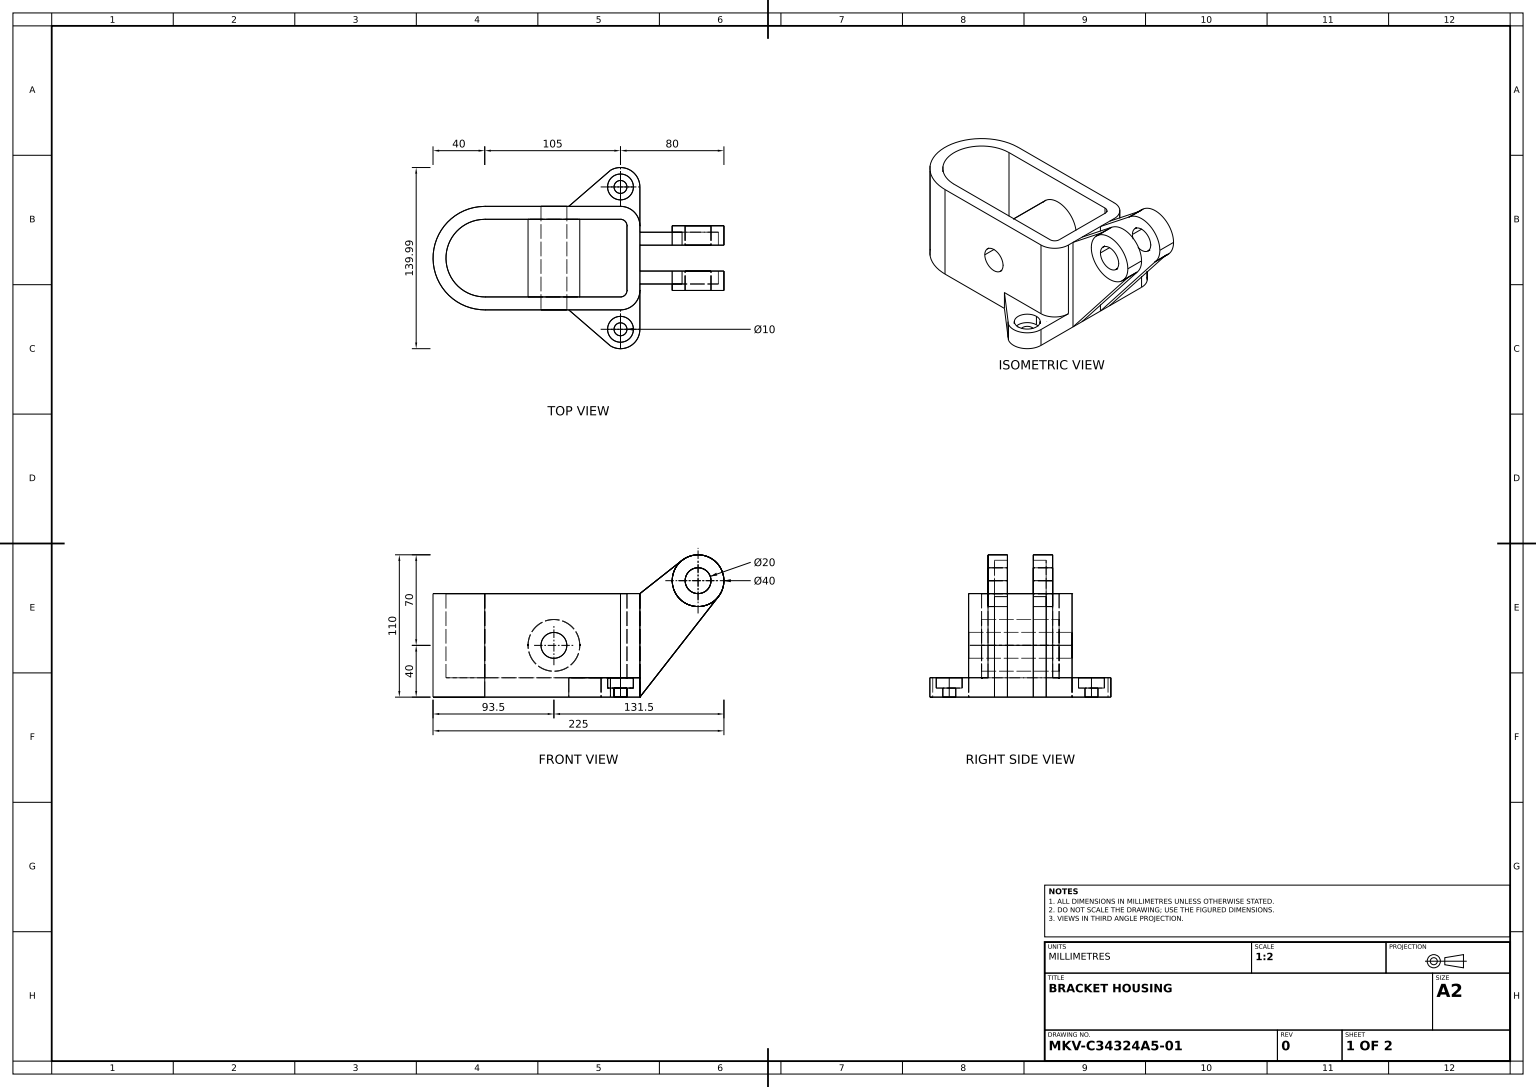
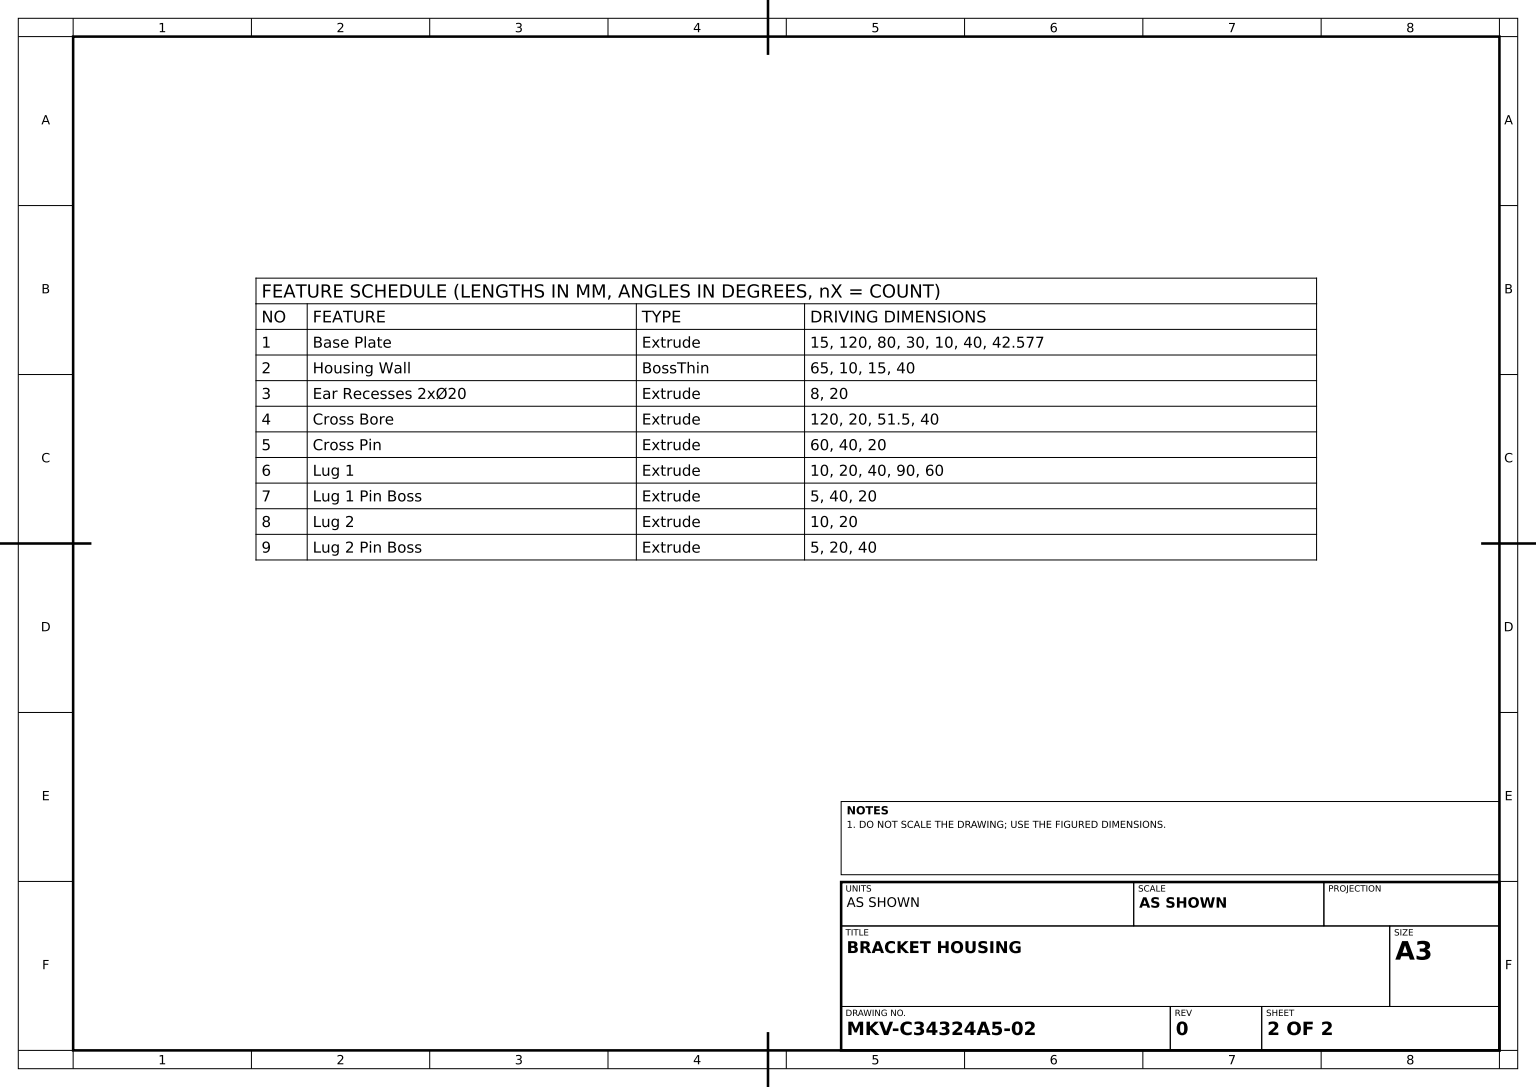
solid
v1 (85,90,20)
v2 (120.753851,77.67863,20)
e1 v1 v2 CIRCLE(AX(P(105,90,20),D(0,0,1),D(1,0,0)),20)
v3 (120.753851,77.67863,10)
e2 v2 v3 LINE
v4 (125,90,10)
e3 v3 v4 CIRCLE(AX(P(105,90,10),D(0,0,1),D(1,0,0)),20)
v5 (125,90,25)
e4 v5 v4 LINE
v6 (85,90,25)
e5 v6 v5 CIRCLE(AX(P(105,90,25),D(0,0,1),D(1,0,0)),20)
e6 v6 v1 LINE
face CYL(AX(P(105,90,20),D(0,0,-1),D(-1,0,0)),20) [e1 e2 e3 -e4 -e5 e6]
v7 (45,15,30)
v8 (50,15,25)
e7 v7 v8 CIRCLE(AX(P(45,15,25),D(0,1,0),D(1,0,0)),5)
v9 (45,80,30)
e8 v9 v7 LINE
v10 (50,80,25)
e9 v9 v10 CIRCLE(AX(P(45,80,25),D(0,1,0),D(1,0,0)),5)
e10 v10 v8 LINE
face CYL(AX(P(45,80,25),D(0,-1,0),D(0,0,-1)),5) rev [-e7 -e8 e9 e10]
v11 (5,15,40)
v12 (5,0,40)
e11 v11 v12 LINE
v13 (37.224741,0,67.827523)
e12 v12 v13 LINE
v14 (37.224741,15,67.827523)
e13 v14 v13 LINE
e14 v11 v14 LINE
face PLANE(AX(P(-17.650842,15,20.439972),D(0.653580385,0,-0.756857107),D(-0.756857107,0,-0.653580385))) rev [e11 e12 -e13 -e14]
v15 (45,0,-50)
v16 (45,0,-60)
e15 v15 v16 CIRCLE(AX(P(45,0,-55),D(0,1,0),D(0,0,1)),5)
e16 v16 v15 CIRCLE(AX(P(45,0,-55),D(0,1,0),D(0,0,1)),5)
v17 (45,0,60)
v18 (45,0,50)
e17 v17 v18 CIRCLE(AX(P(45,0,55),D(0,1,0),D(0,0,1)),5)
e18 v18 v17 CIRCLE(AX(P(45,0,55),D(0,1,0),D(0,0,1)),5)
v19 (-60,0,-40)
v20 (5,0,-40)
e19 v19 v20 LINE
v21 (37.224741,0,-67.827523)
e20 v20 v21 LINE
v22 (45,0,-70)
e21 v22 v21 CIRCLE(AX(P(45,0,-55),D(0,1,0),D(0,0,1)),15)
v23 (60,0,-55)
e22 v23 v22 CIRCLE(AX(P(45,0,-55),D(0,1,0),D(0,0,1)),15)
v24 (60,0,-20)
e23 v24 v23 LINE
v25 (60,0,-10)
e24 v24 v25 LINE
v26 (60,0,10)
e25 v26 v25 LINE
v27 (60,0,20)
e26 v27 v26 LINE
v28 (60,0,55)
e27 v28 v27 LINE
e28 v13 v28 CIRCLE(AX(P(45,0,55),D(0,1,0),D(0,0,1)),15)
v29 (-60,0,40)
e29 v29 v12 LINE
e30 v19 v29 CIRCLE(AX(P(-60,0,0),D(0,1,0),D(0,0,1)),40)
face PLANE(AX(P(0,0,0),D(0,1,0),D(0,0,1))) rev [e15 e16] [e17 e18] [e19 e20 -e21 -e22 -e23 e24 -e25 -e26 -e27 -e28 -e12 -e29 -e30]
v30 (45,7,-45)
v31 (45,15,-45)
e31 v30 v31 LINE
v32 (45,15,-65)
e32 v31 v32 CIRCLE(AX(P(45,15,-55),D(0,1,0),D(0,0,1)),10)
v33 (45,7,-65)
e33 v33 v32 LINE
e34 v30 v33 CIRCLE(AX(P(45,7,-55),D(0,1,0),D(0,0,1)),10)
face CYL(AX(P(45,7,-55),D(0,1,0),D(0,0,1)),10) rev [e31 e32 -e33 -e34]
v34 (95,90,-25)
v35 (115,90,-25)
e35 v34 v35 CIRCLE(AX(P(105,90,-25),D(0,0,-1),D(-1,0,0)),10)
v36 (115,90,-10)
e36 v35 v36 LINE
v37 (95,90,-10)
e37 v36 v37 CIRCLE(AX(P(105,90,-10),D(0,0,1),D(1,0,0)),10)
e38 v34 v37 LINE
face CYL(AX(P(105,90,-20),D(0,0,1),D(1,0,0)),10) rev [e35 e36 e37 -e38]
v38 (3.5,40,40)
v39 (-16.5,40,40)
e39 v38 v39 CIRCLE(AX(P(-6.5,40,40),D(0,0,1),D(1,0,0)),10)
e40 v39 v38 CIRCLE(AX(P(-6.5,40,40),D(0,0,1),D(1,0,0)),10)
v40 (45,15,40)
e41 v11 v40 LINE
v41 (45,80,40)
e42 v41 v40 LINE
v42 (-60,80,40)
e43 v42 v41 LINE
e44 v42 v29 LINE
face PLANE(AX(P(0,15,40),D(0,0,-1),D(-1,0,0))) rev [-e39 -e40] [e29 -e11 e41 -e42 -e43 e44]
v43 (3.5,40,-40)
v44 (-16.5,40,-40)
e45 v43 v44 CIRCLE(AX(P(-6.5,40,-40),D(0,0,-1),D(-1,0,0)),10)
e46 v44 v43 CIRCLE(AX(P(-6.5,40,-40),D(0,0,-1),D(-1,0,0)),10)
v45 (-60,80,-40)
e47 v45 v19 LINE
v46 (45,80,-40)
e48 v46 v45 LINE
v47 (45,15,-40)
e49 v46 v47 LINE
v48 (5,15,-40)
e50 v47 v48 LINE
e51 v48 v20 LINE
face PLANE(AX(P(0,15,-40),D(0,0,-1),D(-1,0,0))) [-e45 -e46] [-e19 -e47 -e48 e49 e50 e51]
v49 (120.753851,77.67863,-10)
v50 (125,90,-10)
e52 v49 v50 CIRCLE(AX(P(105,90,-10),D(0,0,1),D(1,0,0)),20)
v51 (120.753851,77.67863,-20)
e53 v51 v49 LINE
v52 (85,90,-20)
e54 v51 v52 CIRCLE(AX(P(105,90,-20),D(0,0,-1),D(1,0,0)),20)
v53 (85,90,-25)
e55 v53 v52 LINE
v54 (125,90,-25)
e56 v54 v53 CIRCLE(AX(P(105,90,-25),D(0,0,-1),D(-1,0,0)),20)
e57 v54 v50 LINE
face CYL(AX(P(105,90,-20),D(0,0,1),D(1,0,0)),20) [-e52 -e53 e54 -e55 -e56 e57]
v55 (13.5,40,30)
v56 (-26.5,40,30)
e58 v55 v56 CIRCLE(AX(P(-6.5,40,30),D(0,0,1),D(1,0,0)),20)
v57 (13.5,40,-30)
e59 v55 v57 LINE
v58 (-26.5,40,-30)
e60 v57 v58 CIRCLE(AX(P(-6.5,40,-30),D(0,0,1),D(1,0,0)),20)
e61 v56 v58 LINE
face CYL(AX(P(-6.5,40,30),D(0,0,-1),D(-1,0,0)),20) [-e58 e59 e60 -e61]
v59 (45,7,45)
v60 (45,15,45)
e62 v59 v60 LINE
v61 (45,15,65)
e63 v60 v61 CIRCLE(AX(P(45,15,55),D(0,1,0),D(0,0,1)),10)
v62 (45,7,65)
e64 v62 v61 LINE
e65 v59 v62 CIRCLE(AX(P(45,7,55),D(0,1,0),D(0,0,1)),10)
face CYL(AX(P(45,7,55),D(0,1,0),D(0,0,1)),10) rev [e62 e63 -e64 -e65]
v63 (-60,80,-30)
v64 (-60,80,30)
e66 v63 v64 CIRCLE(AX(P(-60,80,0),D(0,1,0),D(1,0,0)),30)
v65 (-60,15,30)
e67 v64 v65 LINE
v66 (-60,15,-30)
e68 v66 v65 CIRCLE(AX(P(-60,15,0),D(0,1,0),D(1,0,0)),30)
e69 v63 v66 LINE
face CYL(AX(P(-60,80,0),D(0,-1,0),D(0,0,-1)),30) rev [e66 e67 -e68 -e69]
v67 (60,80,-10)
e70 v67 v25 LINE
v68 (60,80,10)
e71 v68 v67 LINE
e72 v68 v26 LINE
face PLANE(AX(P(60,15,0),D(-1,0,0),D(0,0,1))) rev [-e70 -e71 e72 e25]
v69 (60,15,-55)
e73 v69 v23 LINE
v70 (60,15,-25)
e74 v70 v69 LINE
v71 (60,80,-25)
e75 v71 v70 LINE
v72 (60,80,-20)
e76 v72 v71 LINE
e77 v72 v24 LINE
face PLANE(AX(P(60,15,0),D(-1,0,0),D(0,0,1))) rev [-e73 -e74 -e75 -e76 e77 e23]
e78 v65 v7 LINE
v73 (50,15,-25)
e79 v8 v73 LINE
v74 (45,15,-30)
e80 v73 v74 CIRCLE(AX(P(45,15,-25),D(0,1,0),D(1,0,0)),5)
e81 v74 v66 LINE
face PLANE(AX(P(0,15,0),D(0,1,0),D(0,0,1))) [e68 e78 e7 e79 e80 e81]
e82 v70 v47 CIRCLE(AX(P(45,15,-25),D(0,1,0),D(0,0,-1)),15)
v75 (45,15,-70)
e83 v69 v75 CIRCLE(AX(P(45,15,-55),D(0,1,0),D(0,0,1)),15)
v76 (37.224741,15,-67.827523)
e84 v75 v76 CIRCLE(AX(P(45,15,-55),D(0,1,0),D(0,0,1)),15)
e85 v48 v76 LINE
e86 v32 v31 CIRCLE(AX(P(45,15,-55),D(0,1,0),D(0,0,1)),10)
face PLANE(AX(P(0,15,0),D(0,1,0),D(0,0,1))) [-e50 -e82 e74 e83 e84 -e85] [-e86 -e32]
v77 (95,90,10)
v78 (115,90,10)
e87 v77 v78 CIRCLE(AX(P(105,90,10),D(0,0,1),D(1,0,0)),10)
v79 (95,90,25)
e88 v79 v77 LINE
v80 (115,90,25)
e89 v79 v80 CIRCLE(AX(P(105,90,25),D(0,0,1),D(1,0,0)),10)
e90 v80 v78 LINE
face CYL(AX(P(105,90,20),D(0,0,-1),D(-1,0,0)),10) rev [-e87 -e88 e89 e90]
e91 v61 v60 CIRCLE(AX(P(45,15,55),D(0,1,0),D(0,0,1)),10)
e92 v62 v59 CIRCLE(AX(P(45,7,55),D(0,1,0),D(0,0,1)),10)
face CYL(AX(P(45,7,55),D(0,1,0),D(0,0,1)),10) rev [e91 -e62 -e92 e64]
v81 (50,80,-25)
e93 v10 v81 LINE
e94 v81 v73 LINE
face PLANE(AX(P(50,80,25),D(-1,0,0),D(0,0,1))) [-e79 -e10 e93 e94]
e95 v71 v46 CIRCLE(AX(P(45,80,-25),D(0,1,0),D(0,0,-1)),15)
e96 v45 v42 CIRCLE(AX(P(-60,80,0),D(0,1,0),D(0,0,1)),40)
v82 (60,80,25)
e97 v41 v82 CIRCLE(AX(P(45,80,25),D(0,1,0),D(0,0,1)),15)
v83 (60,80,20)
e98 v82 v83 LINE
e99 v83 v68 LINE
e100 v72 v67 LINE
v84 (45,80,-30)
e101 v84 v63 LINE
e102 v81 v84 CIRCLE(AX(P(45,80,-25),D(0,1,0),D(1,0,0)),5)
e103 v64 v9 LINE
face PLANE(AX(P(-60,80,0),D(0,1,0),D(0,0,1))) [e76 e95 e48 e96 e43 e97 e98 e99 e71 -e100] [-e66 -e101 -e102 -e93 -e9 -e103]
e104 v26 v3 LINE
v85 (92.620412,105.708145,10)
e105 v68 v85 LINE
e106 v4 v85 CIRCLE(AX(P(105,90,10),D(0,0,1),D(1,0,0)),20)
e107 v78 v77 CIRCLE(AX(P(105,90,10),D(0,0,1),D(1,0,0)),10)
face PLANE(AX(P(0,0,10),D(0,0,1),D(1,0,0))) rev [-e3 -e104 -e72 e105 -e106] [e87 e107]
v86 (45,7,-50)
v87 (45,7,-60)
e108 v86 v87 CIRCLE(AX(P(45,7,-55),D(0,1,0),D(0,0,1)),5)
e109 v87 v16 LINE
e110 v86 v15 LINE
face CYL(AX(P(45,15,-55),D(0,-1,0),D(0,0,-1)),5) rev [e108 e109 -e15 -e110]
v88 (60,15,55)
v89 (60,15,25)
e111 v88 v89 LINE
e112 v40 v89 CIRCLE(AX(P(45,15,25),D(0,1,0),D(0,0,1)),15)
e113 v14 v88 CIRCLE(AX(P(45,15,55),D(0,1,0),D(0,0,1)),15)
face PLANE(AX(P(0,15,0),D(0,1,0),D(0,0,1))) [e111 -e112 -e41 e14 e113] [-e91 -e63]
e114 v87 v86 CIRCLE(AX(P(45,7,-55),D(0,1,0),D(0,0,1)),5)
e115 v33 v30 CIRCLE(AX(P(45,7,-55),D(0,1,0),D(0,0,1)),10)
face PLANE(AX(P(45,7,-55),D(0,1,0),D(0,0,1))) [-e114 -e108] [e34 e115]
face CYL(AX(P(45,80,-25),D(0,-1,0),D(0,0,-1)),15) [-e49 -e95 e75 e82]
e116 v82 v89 LINE
face CYL(AX(P(45,80,25),D(0,-1,0),D(0,0,-1)),15) [-e116 -e97 e42 e112]
e117 v43 v38 LINE
e118 v44 v39 LINE
face CYL(AX(P(-6.5,40,-80),D(0,0,1),D(1,0,0)),10) rev [-e117 e45 e118 e40]
e119 v58 v57 CIRCLE(AX(P(-6.5,40,-30),D(0,0,1),D(1,0,0)),20)
e120 v84 v74 LINE
face PLANE(AX(P(-60,80,-30),D(0,0,1),D(1,0,0))) [-e60 -e119] [e69 -e81 -e120 e101]
e121 v88 v28 LINE
face CYL(AX(P(45,15,55),D(0,-1,0),D(0,0,-1)),15) [e28 -e121 -e113 e13]
face CYL(AX(P(-60,15,0),D(0,-1,0),D(0,0,-1)),40) [e47 e30 -e44 -e96]
v90 (92.620412,105.708145,20)
e122 v83 v90 LINE
e123 v83 v27 LINE
e124 v27 v2 LINE
e125 v90 v1 CIRCLE(AX(P(105,90,20),D(0,0,1),D(1,0,0)),20)
face PLANE(AX(P(0,0,20),D(0,0,1),D(1,0,0))) [-e122 e123 e124 -e1 -e125]
e126 v35 v34 CIRCLE(AX(P(105,90,-25),D(0,0,-1),D(-1,0,0)),10)
e127 v37 v36 CIRCLE(AX(P(105,90,-10),D(0,0,1),D(1,0,0)),10)
face CYL(AX(P(105,90,-20),D(0,0,1),D(1,0,0)),10) rev [-e36 e126 e38 e127]
v91 (45,7,60)
e128 v91 v17 LINE
v92 (45,7,50)
e129 v92 v18 LINE
e130 v92 v91 CIRCLE(AX(P(45,7,55),D(0,1,0),D(0,0,1)),5)
face CYL(AX(P(45,15,55),D(0,-1,0),D(0,0,-1)),5) rev [e128 -e18 -e129 e130]
e131 v91 v92 CIRCLE(AX(P(45,7,55),D(0,1,0),D(0,0,1)),5)
face PLANE(AX(P(45,7,55),D(0,1,0),D(0,0,1))) [e92 e65] [-e130 -e131]
e132 v25 v49 LINE
e133 v24 v51 LINE
face PLANE(AX(P(37.227576,-29.116355,-20),D(0.787692574,-0.616068509,0),D(0.616068509,0.787692574,0))) [e53 -e132 -e24 e133]
e134 v56 v55 CIRCLE(AX(P(-6.5,40,30),D(0,0,1),D(1,0,0)),20)
face PLANE(AX(P(-60,80,30),D(0,0,-1),D(-1,0,0))) [-e78 -e67 e103 e8] [e134 e58]
v93 (92.620412,105.708145,-20)
e135 v93 v72 LINE
e136 v52 v93 CIRCLE(AX(P(105,90,-20),D(0,0,-1),D(1,0,0)),20)
face PLANE(AX(P(0,0,-20),D(0,0,1),D(1,0,0))) rev [-e133 -e77 -e135 -e136 -e54]
face CYL(AX(P(45,15,-55),D(0,-1,0),D(0,0,-1)),5) rev [-e109 e114 e110 -e16]
e137 v5 v6 CIRCLE(AX(P(105,90,25),D(0,0,1),D(1,0,0)),20)
e138 v80 v79 CIRCLE(AX(P(105,90,25),D(0,0,1),D(1,0,0)),10)
face PLANE(AX(P(105,90,25),D(0,0,1),D(1,0,0))) [e137 e5] [-e89 -e138]
face CYL(AX(P(45,80,-25),D(0,-1,0),D(0,0,-1)),5) rev [e120 -e80 -e94 e102]
face CYL(AX(P(45,15,55),D(0,-1,0),D(0,0,-1)),5) rev [-e17 -e128 e131 e129]
face CYL(AX(P(45,7,-55),D(0,1,0),D(0,0,1)),10) rev [e86 -e31 -e115 e33]
e139 v75 v22 LINE
face CYL(AX(P(45,15,-55),D(0,-1,0),D(0,0,-1)),15) [e22 -e139 -e83 e73]
e140 v76 v21 LINE
face PLANE(AX(P(-17.650842,15,-20.439972),D(-0.653580385,0,-0.756857107),D(-0.756857107,0,0.653580385))) [-e20 -e51 e85 e140]
e141 v53 v54 CIRCLE(AX(P(105,90,-25),D(0,0,-1),D(-1,0,0)),20)
face PLANE(AX(P(105,90,-25),D(0,0,-1),D(-1,0,0))) [-e35 -e126] [e141 e56]
face PLANE(AX(P(60,15,0),D(-1,0,0),D(0,0,1))) rev [e116 -e111 e121 e27 -e123 -e98]
e142 v90 v85 LINE
face PLANE(AX(P(-15.903942,20.180109,20),D(-0.618979385,0.785407233,0),D(-0.785407233,-0.618979385,0))) [-e99 e122 e142 -e105]
face CYL(AX(P(105,90,20),D(0,0,-1),D(-1,0,0)),20) [-e6 -e137 e4 e106 -e142 e125]
face CYL(AX(P(-6.5,40,-80),D(0,0,1),D(1,0,0)),10) rev [e117 e39 -e118 e46]
v94 (92.620412,105.708145,-10)
e143 v93 v94 LINE
e144 v50 v94 CIRCLE(AX(P(105,90,-10),D(0,0,1),D(1,0,0)),20)
face CYL(AX(P(105,90,-20),D(0,0,1),D(1,0,0)),20) [e136 e143 -e144 -e57 -e141 e55]
face CYL(AX(P(-6.5,40,30),D(0,0,-1),D(-1,0,0)),20) [e119 -e59 -e134 e61]
e145 v94 v67 LINE
face PLANE(AX(P(0,0,-10),D(0,0,1),D(1,0,0))) [-e127 -e37] [e70 e132 e52 e144 e145]
face CYL(AX(P(105,90,20),D(0,0,-1),D(-1,0,0)),10) rev [e138 e88 -e107 -e90]
face PLANE(AX(P(-15.903942,20.180109,-20),D(-0.618979385,0.785407233,0),D(-0.785407233,-0.618979385,0))) [-e145 -e143 e135 e100]
face CYL(AX(P(45,15,-55),D(0,-1,0),D(0,0,-1)),15) [e139 e21 -e140 -e84]
face PLANE(AX(P(37.227576,-29.116355,20),D(-0.787692574,0.616068509,0),D(-0.616068509,-0.787692574,0))) rev [-e124 e26 e104 -e2]
